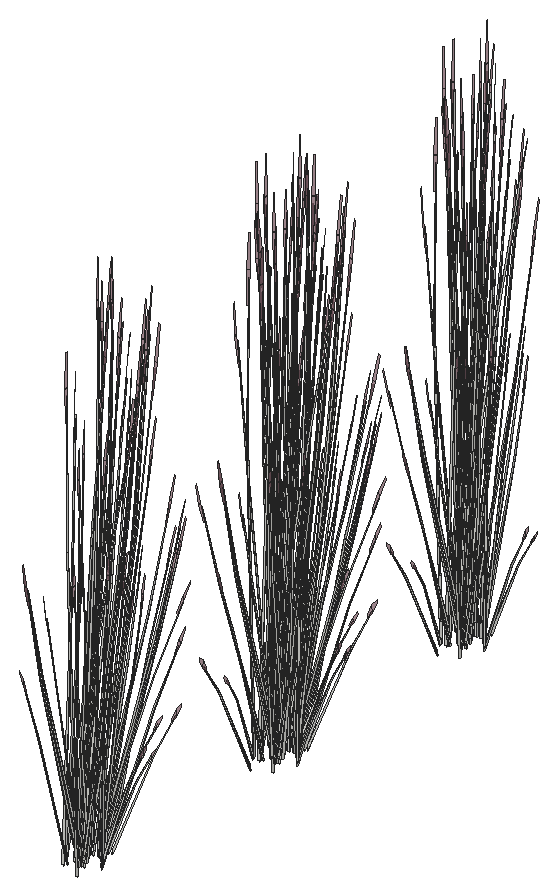
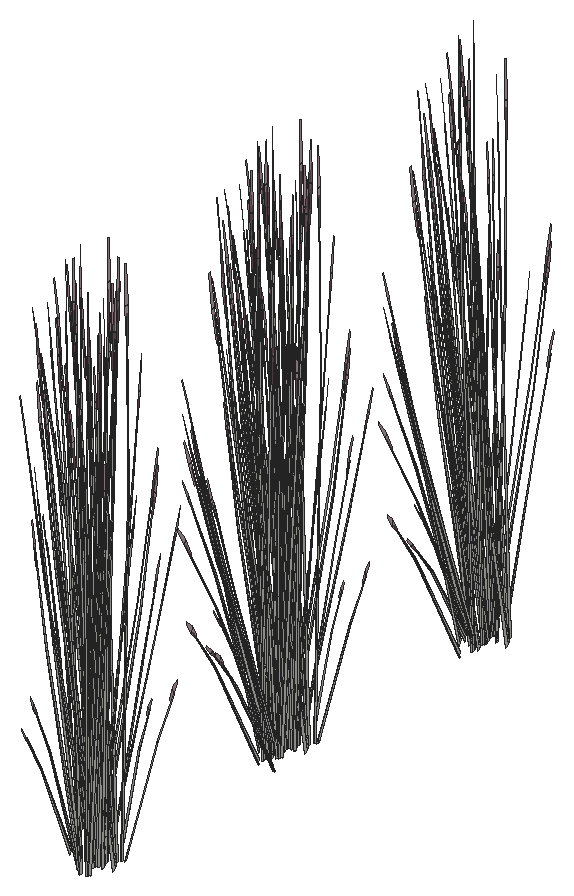
# SketchUp Ruby script. Lengths in inches.
U = 1.inch
M = Sketchup.active_model
def pt(a) = Geom::Point3d.new(a.map { |v| v * U })
def face(e, loops, mat)
  f = e.add_face(loops[0].map { |a| pt(a) })
  loops[1..].each { |l| e.add_face(l.map { |a| pt(a) }).erase! }
  f.material = f.back_material = mat if mat
  f
end
# faces: each face lists its corners as indices into pts; further lists are holes
def faces(e, pts, list, mat = nil) = list.each { |f| face(e, (f[0].is_a?(Array) ? f : [f]).map { |l| l.map { |i| pts[i] } }, mat) }
# xy, xz, yz: faces in a plane at the given z, y or x. An outline is a flat list of corners, or four numbers for a rectangle; further outlines are holes
def ring(l) = l.size == 4 ? [[l[0], l[1]], [l[2], l[1]], [l[2], l[3]], [l[0], l[3]]] : l.each_slice(2).to_a
def flat(e, list, mat, &to3) = list.each { |f| face(e, (f[0].is_a?(Array) ? f : [f]).map { |l| ring(l).map { |u, v| to3.(u, v) } }, mat) }
def xy(e, z, list, mat = nil) = flat(e, list, mat) { |x, y| [x, y, z] }
def xz(e, y, list, mat = nil) = flat(e, list, mat) { |x, z| [x, y, z] }
def yz(e, x, list, mat = nil) = flat(e, list, mat) { |y, z| [x, y, z] }
def lines(e, pts, list) = list.each { |a, b| e.add_line(pt(pts[a]), pt(pts[b])) }
# prism: a flat outline (further loops are holes) pulled along v
def prism(e, loops, v, mat = nil)
  f = face(e, loops, mat); d = Geom::Vector3d.new(v.map { |x| x * U })
  f.pushpull(f.normal.samedirection?(d) ? d.length : -d.length)
end
def box(e, o, s, mat = nil) = prism(e, [[o, [o[0] + s[0], o[1], o[2]], [o[0] + s[0], o[1] + s[1], o[2]], [o[0], o[1] + s[1], o[2]]]], [0, 0, s[2]], mat)
def at(x, y, z, deg = 0) = Geom::Transformation.translation(pt([x, y, z])) * Geom::Transformation.rotation(ORIGIN, Z_AXIS, deg.degrees)
def axes(o, x, y, z) = Geom::Transformation.new([*x, 0, *y, 0, *z, 0, *pt(o).to_a, 1])
def part(name) = M.definitions.add(name)
# library, detail: a bought-in or finely detailed component or shape, given as its bounding box
def library(name, o, s) = part(name).tap { |d| box(d.entities, o, s) }
def detail(e, o, s) = box(e.add_group.entities, o, s)
def put(e, d, t, mat = nil) = e.add_instance(d, t).tap { |i| i.material = mat if mat }
def group(e, t, mat = nil) = e.add_group.tap { |g| g.transformation = t; g.material = mat if mat }.entities
root = M.entities
M.materials.add("LightPink_Translucent").color = [144, 107, 117]
M.materials["LightPink_Translucent"].alpha = 0.75
c1 = part("blade")
p = [[2.15,0.21,22],[0,0.17,0],[0.09,0.45,0],[2.18,0.31,22],[2.29,0.31,22],[0.38,0.45,0],
  [2.48,0.24,33],[2.49,0.24,33],[2.48,0.22,33]]
faces(c1.entities,p,[[0,1,2,3],[4,5,2,3],[6,3,4,7],[8,0,3,6]])
c2 = part("seeds")
p = [[0.3,-0.1,1.38],[-0.01,-0.03,1.59],[-0.01,-0.03,0.03],[0.14,-0.07,-0.07],[0.29,-0.03,3],[0.15,0.01,3.11]]
faces(c2.entities,p,[[0,1,2,3],[1,0,4,5]],"LightPink_Translucent")
c3 = part("blade with seeds")
put(c3.entities,c1,at(0,0,0))
put(c3.entities,c2,axes([2.4,0.25,30.99],[1.5799,-0.05474,1.17369],[-0.12525,1.92788,0.29478],[-0.07173,-0.02425,1.56792]))
put(root,c3,axes([431.59,18.82,0.23],[-0.10696,0.11169,1.22981],[-0.32033,-0.19549,-0.26449],[0.05938,-0.24312,0.52581]))
put(root,c3,axes([431.85,19.65,2.28],[0.00979,-0.51041,-0.61099],[0.4123,0.03428,0.07373],[0.04351,-0.21623,0.8643]))
put(root,c3,axes([431.77,19.48,2.03],[-0.26937,-0.37076,-0.43945],[0.28456,-0.3247,-0.34039],[0.04099,-0.18838,0.84085]))
put(root,c3,axes([432.02,19.34,1.89],[0.2546,-0.29052,-0.30456],[0.24101,0.33173,0.39319],[0.03667,-0.16855,0.75234]))
put(root,c3,axes([432.34,19.17,-0.72],[-0.05632,-0.04347,1.51654],[-0.14467,-0.48565,-0.23168],[0.09759,-0.13179,0.25832]))
put(root,c3,axes([432.34,20.54,2.28],[0.19655,-0.43539,-0.61099],[0.34443,0.30942,0.07373],[0.11736,-0.15774,0.8643]))
put(root,c3,axes([432.33,20.33,2.03],[-0.09666,-0.50384,-0.43945],[0.36608,-0.08814,-0.34039],[0.10491,-0.13533,0.84085]))
put(root,c3,axes([430.53,19.18,-0.26],[0.35217,-0.2759,-0.427],[0.2105,0.49473,0],[0.08021,-0.06284,1.35453]))
put(root,c3,axes([432.625,20.14,0.23],[-0.13443,-0.01634,1.22981],[-0.13772,-0.43844,-0.26449],[0.16514,-0.12403,0.52581]))
put(root,c3,axes([430.95,20.31,-0.23],[0.25345,-0.41475,-0.53624],[0.31485,0.37608,-0.14074],[0.10156,-0.10346,1.18365]))
put(root,c3,axes([432.78,19.33,0.38],[-0.12533,0.28089,0.9878],[-0.10773,-0.37739,0.72577],[0.10352,-0.09457,0.21757]))
put(root,c3,axes([432.6,20.39,1.89],[0.32754,-0.07886,-0.30456],[0.08649,0.45081,0.39319],[0.09386,-0.12109,0.75234]))
put(root,c3,axes([430.68,20.8,0.29],[-0.04385,-0.62963,-0.25022],[0.45669,-0.03807,-0.43002],[0.08042,-0.08387,1.37348]))
put(root,c3,axes([430.62,19.4,-0.26],[0.35106,0.13653,-0.26641],[-0.08839,0.48081,0.26641],[0.07077,-0.05545,1.19518]))
put(root,c3,axes([432.5,21.45,2.03],[0.10194,-0.50193,-0.43945],[0.34951,0.17204,-0.34039],[0.14072,-0.04602,0.84085]))
put(root,c3,axes([431.95,19.41,0.04],[0.23526,-0.55293,0],[0.3936,0.30836,-0.44382],[0.08964,0.07023,1.40792]))
put(root,c3,axes([432.875,21.59,-0.3],[-0.24235,0.06622,1.21762],[-0.03858,-0.5271,0.0697],[0.16974,-0.07978,0.69287]))
put(root,c3,axes([433.31,21.125,-0.06],[-0.23329,-0.35284,-0.05579],[0.2555,-0.3233,-0.25298],[0.0724,-0.02276,0.83441]))
put(root,c3,axes([431.74,19.7,0.13],[-0.35217,-0.2759,0.427],[0.2105,-0.49473,0],[0.08021,0.06284,1.35453]))
put(root,c3,axes([432.43,21.63,2.28],[0.33065,-0.2437,-0.61099],[0.18427,0.50165,0.07373],[0.15976,-0.05699,0.8643]))
put(root,c3,axes([430.25,20.39,-0.63],[-0.37038,0.22092,1.10879],[-0.11789,-0.63387,0.43083],[0.22743,0.01055,1.26112]))
put(root,c3,axes([431.24,20.55,0.25],[0.07259,-0.49245,0.12452],[0.35466,0.08548,-0.35559],[0.06454,0.05057,1.09]))
put(root,c3,axes([433.14,21.25,-0.72],[-0.01967,-0.08377,1.51654],[0.1364,-0.49004,-0.23168],[0.13759,-0.00705,0.25832]))
put(root,c3,axes([431.09,20.68,0.34],[-0.22605,-0.46315,0.38476],[0.34239,-0.32614,-0.18517],[0.07315,0.05731,1.23533]))
put(root,c3,axes([431.2,20.71,0.29],[0.37992,-0.36634,-0.25022],[0.25264,0.51764,-0.43002],[0.09374,0.05257,1.37348]))
put(root,c3,axes([432.71,21.68,1.89],[0.31272,0.15393,-0.30456],[-0.09121,0.44909,0.39319],[0.1259,-0.04118,0.75234]))
put(root,c3,axes([432.16,19.74,-0.26],[0.35217,0.2759,-0.427],[-0.2105,0.49473,0],[0.08021,0.06284,1.35453]))
put(root,c3,axes([431.49,21.31,-0.1],[0.42099,0,0],[0,0.57126,0],[0,0,1.5343]))
put(root,c3,axes([432.0625,19.95,-0.26],[0.08839,0.48081,-0.26641],[-0.35106,0.13653,0.26641],[0.07077,0.05545,1.19518]))
put(root,c3,axes([431.36,21.02,0.05],[-0.4756,-0.11626,0.42311],[0.09679,-0.6566,0.16603],[0.0695,0.0634,1.46899]))
put(root,c3,axes([431.4375,22.58,-0.12],[0.39505,-0.18722,-0.1651],[0.13882,0.53931,0.00007],[0.04361,-0.02069,1.49552]))
put(root,c3,axes([431.48,21.56,-0.1],[0.26266,0.35642,0],[-0.26266,0.35642,0],[0,0,1.45569]))
put(root,c3,axes([431.65,20.8,-0.23],[0.39143,0.09047,-0.53624],[-0.0826,0.55804,-0.14074],[0.11681,0.06762,1.18365]))
put(root,c3,axes([433.38,21.77,0.38],[-0.23249,0.0911,0.9878],[0.10944,-0.37648,0.72577],[0.12334,0.02576,0.21757]))
put(root,c3,axes([431.48,21.14,0.34],[0.18257,-0.49721,0.38476],[0.37935,0.23929,-0.18517],[0,0.11462,1.23533]))
put(root,c3,axes([431.45,20.97,-0.1],[0.22605,0.46315,-0.38476],[-0.34239,0.32614,0.18517],[0.07315,0.05731,1.23533]))
put(root,c3,axes([432.4375,21.42,0.13],[0,-0.5518,0.427],[0.42099,0,0],[0,0.12568,1.35453]))
put(root,c3,axes([431.64,21.26,0.25],[0.35059,-0.16092,0.12452],[0.12277,0.45952,-0.35559],[0,0.10113,1.09]))
put(root,c3,axes([432.94,22.375,0.23],[-0.09062,-0.13571,1.22981],[0.11791,-0.44895,-0.26449],[0.18335,0.06082,0.52581]))
put(root,c3,axes([431.32,22.87,-0.1],[0.37935,0.24773,0],[-0.18257,0.51475,0],[0,0,1.5046]))
put(root,c3,axes([432.11,22.65,2.28],[0.37615,0.01329,-0.61099],[-0.02526,0.55946,0.07373],[0.15935,0.05904,0.8643]))
put(root,c3,axes([432.72,21.51,0.04],[0.47052,0,0],[0,0.61671,-0.44382],[0,0.14046,1.40792]))
put(root,c3,axes([431.52,21.29,0.29],[0.42377,0.26329,-0.25022],[-0.20405,0.55571,-0.43002],[0.01332,0.13644,1.37348]))
put(root,c3,axes([432.34,22.88,1.89],[0.2141,0.34548,-0.30456],[-0.24447,0.32704,0.39319],[0.12421,0.04976,0.75234]))
put(root,c3,axes([432.4375,21.92,-0.26],[-0.26266,0.34428,-0.26641],[-0.26266,-0.34428,0.26641],[0,0.11089,1.19518]))
put(root,c3,axes([432.62,21.93,-0.26],[0,0.5518,-0.427],[-0.42099,0,0],[0,0.12568,1.35453]))
put(root,c3,axes([432.08,23.08,0.38],[-0.21187,-0.15866,0.9878],[0.27357,-0.16121,0.72577],[0.07379,0.13656,0.21757]))
put(root,c3,axes([432.14,23.67,-0.72],[0.02741,-0.07966,1.51654],[0.34514,-0.23462,-0.23168],[0.10464,0.12143,0.25832]))
put(root,c3,axes([431.6875,21.86,-0.2],[0.13798,0.50522,-0.59522],[-0.39745,0.18195,-0.15622],[0.01525,0.17108,1.31385]))
put(root,c3,axes([431.61,23.3,2.03],[0.37131,-0.13117,-0.43945],[0.06495,0.49674,-0.34039],[0.09973,0.14235,0.84085]))
put(root,c3,axes([432.12,23.8,0.29],[-0.2413,-0.01731,0.90352],[0.15935,-0.36755,0.49885],[0.09532,0.13058,0.70873]))
put(root,c3,axes([431.33,22.91,0.23],[0.00664,-0.18292,1.22981],[0.31732,-0.20432,-0.26449],[0.09796,0.21893,0.52581]))
put(root,c3,axes([430.78,23.53,2.03],[0.3699,0.13833,-0.43945],[-0.12679,0.47426,-0.34039],[0.03392,0.19095,0.84085]))
put(root,c3,axes([433.22,41.86,0.23],[-0.10696,0.11169,1.22981],[-0.32033,-0.19549,-0.26449],[0.05938,-0.24312,0.52581]))
put(root,c3,axes([432.43,41.26,-0.72],[-0.06312,0.01988,1.51654],[-0.34903,-0.22379,-0.23168],[0.00586,-0.18666,0.25832]))
put(root,c3,axes([433.48,42.69,2.28],[0.00979,-0.51041,-0.61099],[0.4123,0.03428,0.07373],[0.04351,-0.21623,0.8643]))
put(root,c3,axes([432.77,41.87,1.89],[0.11344,-0.42434,-0.30456],[0.33096,0.12377,0.39319],[-0.03035,-0.17085,0.75234]))
put(root,c3,axes([432.83,40.97,0.38],[0.04827,0.32177,0.9878],[-0.26778,-0.17821,0.72577],[0.02882,-0.16476,0.21757]))
put(root,c3,axes([433.4,42.52,2.03],[-0.26937,-0.37076,-0.43945],[0.28456,-0.3247,-0.34039],[0.04099,-0.18838,0.84085]))
put(root,c3,axes([433.65,42.38,1.89],[0.2546,-0.29052,-0.30456],[0.24101,0.33173,0.39319],[0.03667,-0.16855,0.75234]))
put(root,c3,axes([433.97,42.21,-0.72],[-0.05632,-0.04347,1.51654],[-0.14467,-0.48565,-0.23168],[0.09759,-0.13179,0.25832]))
put(root,c3,axes([433.97,43.58,2.28],[0.19655,-0.43539,-0.61099],[0.34443,0.30942,0.07373],[0.11736,-0.15774,0.8643]))
put(root,c3,axes([431.84,42.31,0.04],[-0.23526,-0.55293,0],[0.3936,-0.30836,-0.44382],[0.08964,-0.07023,1.40792]))
put(root,c3,axes([433.96,43.375,2.03],[-0.09666,-0.50384,-0.43945],[0.36608,-0.08814,-0.34039],[0.10491,-0.13533,0.84085]))
put(root,c3,axes([432.16,42.22,-0.26],[0.35217,-0.2759,-0.427],[0.2105,0.49473,0],[0.08021,-0.06284,1.35453]))
put(root,c3,axes([434.25,43.18,0.23],[-0.13443,-0.01634,1.22981],[-0.13772,-0.43844,-0.26449],[0.16514,-0.12403,0.52581]))
put(root,c3,axes([432.58,43.36,-0.23],[0.25345,-0.41475,-0.53624],[0.31485,0.37608,-0.14074],[0.10156,-0.10346,1.18365]))
put(root,c3,axes([434.41,42.37,0.38],[-0.12533,0.28089,0.9878],[-0.10773,-0.37739,0.72577],[0.10352,-0.09457,0.21757]))
put(root,c3,axes([434.23,43.43,1.89],[0.32754,-0.07886,-0.30456],[0.08649,0.45081,0.39319],[0.09386,-0.12109,0.75234]))
put(root,c3,axes([432.14,44.08,-0.1],[0.18257,-0.49721,-0.38476],[0.37935,0.23929,0.18517],[0,-0.11462,1.23533]))
put(root,c3,axes([432.31,43.84,0.29],[-0.04385,-0.62963,-0.25022],[0.45669,-0.03807,-0.43002],[0.08042,-0.08387,1.37348]))
put(root,c3,axes([432.25,42.44,-0.26],[0.35106,0.13653,-0.26641],[-0.08839,0.48081,0.26641],[0.07077,-0.05545,1.19518]))
put(root,c3,axes([432.37,44.33,0.09],[0.42398,0.26744,0.20696],[-0.20405,0.55571,0.43002],[0,-0.1281,1.38067]))
put(root,c3,axes([432.23,43.96,0.34],[-0.40861,0.03406,0.38476],[-0.03695,-0.56543,-0.18517],[0.07315,-0.05731,1.23533]))
put(root,c3,axes([434.13,44.49,2.03],[0.10194,-0.50193,-0.43945],[0.34951,0.17204,-0.34039],[0.14072,-0.04602,0.84085]))
put(root,c3,axes([433.58,42.45,0.04],[0.23526,-0.55293,0],[0.3936,0.30836,-0.44382],[0.08964,0.07023,1.40792]))
put(root,c3,axes([432.22,44.16,0.03],[0.1636,0.61702,0.39349],[-0.46745,0.21456,0.15441],[0.00571,-0.11338,1.36617]))
put(root,c3,axes([434.5,44.63,-0.3],[-0.24235,0.06622,1.21762],[-0.03858,-0.5271,0.0697],[0.16974,-0.07978,0.69287]))
put(root,c3,axes([434.94,44.17,-0.06],[-0.23329,-0.35284,-0.05579],[0.2555,-0.3233,-0.25298],[0.0724,-0.02276,0.83441]))
put(root,c3,axes([432.8,44.21,-0.1],[0,-0.63847,0],[0.47052,0,0],[0,0,1.54332]))
put(root,c3,axes([433.375,42.74,0.13],[-0.35217,-0.2759,0.427],[0.2105,-0.49473,0],[0.08021,0.06284,1.35453]))
put(root,c3,axes([434.0625,44.68,2.28],[0.33065,-0.2437,-0.61099],[0.18427,0.50165,0.07373],[0.15976,-0.05699,0.8643]))
put(root,c3,axes([432.58,43.8125,0.03],[-0.312,0.50076,0.39349],[-0.37066,-0.44204,0.15441],[0.07522,-0.04998,1.36617]))
put(root,c3,axes([432.92,44.71,-0.02],[-0.35001,-0.47494,-0.05273],[0.35022,-0.47523,0],[-0.01222,-0.01659,1.50991]))
put(root,c3,axes([432.04,42.99,0.13],[-0.1087,0.54839,0.15172],[-0.39778,-0.15519,0.30174],[0.06871,-0.00267,1.3795]))
put(root,c3,axes([431.875,43.43,-0.63],[-0.37038,0.22092,1.10879],[-0.11789,-0.63387,0.43083],[0.22743,0.01055,1.26112]))
put(root,c3,axes([432.87,43.6,0.25],[0.07259,-0.49245,0.12452],[0.35466,0.08548,-0.35559],[0.06454,0.05057,1.09]))
put(root,c3,axes([434.77,44.29,-0.72],[-0.01967,-0.08377,1.51654],[0.1364,-0.49004,-0.23168],[0.13759,-0.00705,0.25832]))
put(root,c3,axes([432.72,43.73,0.34],[-0.22605,-0.46315,0.38476],[0.34239,-0.32614,-0.18517],[0.07315,0.05731,1.23533]))
put(root,c3,axes([432,45.82,0.13],[0.40434,-0.14646,0.15172],[0.09984,0.54504,0.30174],[-0.03606,-0.07941,1.3795]))
put(root,c3,axes([432.83,43.76,0.29],[0.37992,-0.36634,-0.25022],[0.25264,0.51764,-0.43002],[0.09374,0.05257,1.37348]))
put(root,c3,axes([434.34,44.72,1.89],[0.31272,0.15393,-0.30456],[-0.09121,0.44909,0.39319],[0.1259,-0.04118,0.75234]))
put(root,c3,axes([433.79,42.78,-0.26],[0.35217,0.2759,-0.427],[-0.2105,0.49473,0],[0.08021,0.06284,1.35453]))
put(root,c3,axes([433.12,44.36,-0.1],[0.42099,0,0],[0,0.57126,0],[0,0,1.5343]))
put(root,c3,axes([433.24,43.02,0.13],[-0.40434,0.14646,0.15172],[-0.09984,-0.54504,0.30174],[0.03606,0.07941,1.3795]))
put(root,c3,axes([433.69,42.99,-0.26],[0.08839,0.48081,-0.26641],[-0.35106,0.13653,0.26641],[0.07077,0.05545,1.19518]))
put(root,c3,axes([432.99,44.07,0.05],[-0.4756,-0.11626,0.42311],[0.09679,-0.6566,0.16603],[0.0695,0.0634,1.46899]))
put(root,c3,axes([432.61,45.6875,-0.1],[-0.12277,-0.47573,0],[0.35059,-0.1666,0],[0,0,1.32759]))
put(root,c3,axes([433.07,45.62,-0.12],[0.39505,-0.18722,-0.1651],[0.13882,0.53931,0.00007],[0.04361,-0.02069,1.49552]))
put(root,c3,axes([433.2,45.85,0.13],[0.1087,-0.54839,0.15172],[0.39778,0.15519,0.30174],[-0.06871,0.00267,1.3795]))
put(root,c3,axes([433.11,44.6,-0.1],[0.26266,0.35642,0],[-0.26266,0.35642,0],[0,0,1.45569]))
put(root,c3,axes([433.82,44.45,0.13],[-0.29564,-0.40194,0.15172],[0.29793,-0.38985,0.30174],[-0.03265,0.08208,1.3795]))
put(root,c3,axes([433.28,43.84,-0.23],[0.39143,0.09047,-0.53624],[-0.0826,0.55804,-0.14074],[0.11681,0.06762,1.18365]))
put(root,c3,axes([435.01,44.8125,0.38],[-0.23249,0.0911,0.9878],[0.10944,-0.37648,0.72577],[0.12334,0.02576,0.21757]))
put(root,c3,axes([432.52,45.9,-0.11],[-0.37935,-0.24773,0],[0.18257,-0.51475,0],[0,0,1.39928]))
put(root,c3,axes([433.11,44.18,0.34],[0.18257,-0.49721,0.38476],[0.37935,0.23929,-0.18517],[0,0.11462,1.23533]))
put(root,c3,axes([433.04,44.47,-0.03],[0,0.63816,-0.04848],[-0.47052,0,0],[0,0.02005,1.54256]))
put(root,c3,axes([433.07,44.02,-0.1],[0.22605,0.46315,-0.38476],[-0.34239,0.32614,0.18517],[0.07315,0.05731,1.23533]))
put(root,c3,axes([434.07,44.46,0.13],[0,-0.5518,0.427],[0.42099,0,0],[0,0.12568,1.35453]))
put(root,c3,axes([433.01,44.875,0.34],[0.40861,-0.03406,0.38476],[0.03695,0.56543,-0.18517],[-0.07315,0.05731,1.23533]))
put(root,c3,axes([433.27,44.3,0.25],[0.35059,-0.16092,0.12452],[0.12277,0.45952,-0.35559],[0,0.10113,1.09]))
put(root,c3,axes([434.57,45.42,0.23],[-0.09062,-0.13571,1.22981],[0.11791,-0.44895,-0.26449],[0.18335,0.06082,0.52581]))
put(root,c3,axes([432.95,45.91,-0.1],[0.37935,0.24773,0],[-0.18257,0.51475,0],[0,0,1.5046]))
put(root,c3,axes([433.02,45.12,0.25],[0.278,0.33153,0.12452],[-0.23189,0.37404,-0.35559],[-0.06454,0.05057,1.09]))
put(root,c3,axes([433.74,45.69,2.28],[0.37615,0.01329,-0.61099],[-0.02526,0.55946,0.07373],[0.15935,0.05904,0.8643]))
put(root,c3,axes([433.32,46.14,0.13],[0.35217,-0.2759,0.427],[0.2105,0.49473,0],[-0.08021,0.06284,1.35453]))
put(root,c3,axes([432.81,45.7,-0.03],[0.1636,0.63392,-0.05171],[-0.46745,0.22213,0],[0.00571,0.02214,1.48069]))
put(root,c3,axes([434.35,44.56,0.04],[0.47052,0,0],[0,0.61671,-0.44382],[0,0.14046,1.40792]))
put(root,c3,axes([434.17,44.87,-0.11],[-0.47029,-0.00441,-0.0428],[0,-0.61671,0.42951],[-0.01478,0.14039,1.36183]))
put(root,c3,axes([433.15,44.34,0.29],[0.42377,0.26329,-0.25022],[-0.20405,0.55571,-0.43002],[0.01332,0.13644,1.37348]))
put(root,c3,axes([433.97,45.92,1.89],[0.2141,0.34548,-0.30456],[-0.24447,0.32704,0.39319],[0.12421,0.04976,0.75234]))
put(root,c3,axes([434.07,44.96,-0.26],[-0.26266,0.34428,-0.26641],[-0.26266,-0.34428,0.26641],[0,0.11089,1.19518]))
put(root,c3,axes([433.1,44.75,-0.1],[-0.18257,0.49721,-0.38476],[-0.37935,-0.23929,0.18517],[0,0.11462,1.23533]))
put(root,c3,axes([433.11,46.17,0],[0.47108,0.17935,0.2645],[-0.11785,0.64108,-0.31383],[-0.07797,0.08023,1.41801]))
put(root,c3,axes([434.25,44.97,-0.26],[0,0.5518,-0.427],[-0.42099,0,0],[0,0.12568,1.35453]))
put(root,c3,axes([433.71,46.12,0.38],[-0.21187,-0.15866,0.9878],[0.27357,-0.16121,0.72577],[0.07379,0.13656,0.21757]))
put(root,c3,axes([433.4,46.52,0.04],[0.23526,0.55293,0],[-0.3936,0.30836,-0.44382],[-0.08964,0.07023,1.40792]))
put(root,c3,axes([433.77,46.71,-0.72],[0.02741,-0.07966,1.51654],[0.34514,-0.23462,-0.23168],[0.10464,0.12143,0.25832]))
put(root,c3,axes([433.32,44.9,-0.2],[0.13798,0.50522,-0.59522],[-0.39745,0.18195,-0.15622],[0.01525,0.17108,1.31385]))
put(root,c3,axes([433.24,46.34,2.03],[0.37131,-0.13117,-0.43945],[0.06495,0.49674,-0.34039],[0.09973,0.14235,0.84085]))
put(root,c3,axes([433.75,46.84,0.29],[-0.2413,-0.01731,0.90352],[0.15935,-0.36755,0.49885],[0.09532,0.13058,0.70873]))
put(root,c3,axes([432.96,45.95,0.23],[0.00664,-0.18292,1.22981],[0.31732,-0.20432,-0.26449],[0.09796,0.21893,0.52581]))
put(root,c3,axes([432.16,46.69,-0.72],[0.0609,-0.03003,1.51654],[0.36632,0.16527,-0.23168],[0.01071,0.18627,0.25832]))
put(root,c3,axes([432.41,46.57,2.03],[0.3699,0.13833,-0.43945],[-0.12679,0.47426,-0.34039],[0.03392,0.19095,0.84085]))
put(root,c3,axes([432.24,46.86,1.89],[-0.11344,0.42434,-0.30456],[-0.33096,-0.12377,0.39319],[0.03035,0.17085,0.75234]))
put(root,c3,axes([432.28,46.48,2.28],[0.17959,0.44867,-0.61099],[-0.36969,0.25004,0.07373],[0.042,0.21679,0.8643]))
put(root,c3,axes([433.22,65.86,0.23],[-0.10696,0.11169,1.22981],[-0.32033,-0.19549,-0.26449],[0.05938,-0.24312,0.52581]))
put(root,c3,axes([432.43,65.26,-0.72],[-0.06312,0.01988,1.51654],[-0.34903,-0.22379,-0.23168],[0.00586,-0.18666,0.25832]))
put(root,c3,axes([433.48,66.69,2.28],[0.00979,-0.51041,-0.61099],[0.4123,0.03428,0.07373],[0.04351,-0.21623,0.8643]))
put(root,c3,axes([432.77,65.87,1.89],[0.11344,-0.42434,-0.30456],[0.33096,0.12377,0.39319],[-0.03035,-0.17085,0.75234]))
put(root,c3,axes([432.83,64.97,0.38],[0.04827,0.32177,0.9878],[-0.26778,-0.17821,0.72577],[0.02882,-0.16476,0.21757]))
put(root,c3,axes([433.4,66.52,2.03],[-0.26937,-0.37076,-0.43945],[0.28456,-0.3247,-0.34039],[0.04099,-0.18838,0.84085]))
put(root,c3,axes([433.65,66.38,1.89],[0.2546,-0.29052,-0.30456],[0.24101,0.33173,0.39319],[0.03667,-0.16855,0.75234]))
put(root,c3,axes([433.97,66.21,-0.72],[-0.05632,-0.04347,1.51654],[-0.14467,-0.48565,-0.23168],[0.09759,-0.13179,0.25832]))
put(root,c3,axes([433.97,67.58,2.28],[0.19655,-0.43539,-0.61099],[0.34443,0.30942,0.07373],[0.11736,-0.15774,0.8643]))
put(root,c3,axes([431.84,66.31,0.04],[-0.23526,-0.55293,0],[0.3936,-0.30836,-0.44382],[0.08964,-0.07023,1.40792]))
put(root,c3,axes([433.96,67.375,2.03],[-0.09666,-0.50384,-0.43945],[0.36608,-0.08814,-0.34039],[0.10491,-0.13533,0.84085]))
put(root,c3,axes([432.16,66.22,-0.26],[0.35217,-0.2759,-0.427],[0.2105,0.49473,0],[0.08021,-0.06284,1.35453]))
put(root,c3,axes([434.25,67.18,0.23],[-0.13443,-0.01634,1.22981],[-0.13772,-0.43844,-0.26449],[0.16514,-0.12403,0.52581]))
put(root,c3,axes([432.58,67.36,-0.23],[0.25345,-0.41475,-0.53624],[0.31485,0.37608,-0.14074],[0.10156,-0.10346,1.18365]))
put(root,c3,axes([434.41,66.37,0.38],[-0.12533,0.28089,0.9878],[-0.10773,-0.37739,0.72577],[0.10352,-0.09457,0.21757]))
put(root,c3,axes([434.23,67.43,1.89],[0.32754,-0.07886,-0.30456],[0.08649,0.45081,0.39319],[0.09386,-0.12109,0.75234]))
put(root,c3,axes([432.14,68.08,-0.1],[0.18257,-0.49721,-0.38476],[0.37935,0.23929,0.18517],[0,-0.11462,1.23533]))
put(root,c3,axes([432.31,67.84,0.29],[-0.04385,-0.62963,-0.25022],[0.45669,-0.03807,-0.43002],[0.08042,-0.08387,1.37348]))
put(root,c3,axes([432.25,66.44,-0.26],[0.35106,0.13653,-0.26641],[-0.08839,0.48081,0.26641],[0.07077,-0.05545,1.19518]))
put(root,c3,axes([432.37,68.33,0.09],[0.42398,0.26744,0.20696],[-0.20405,0.55571,0.43002],[0,-0.1281,1.38067]))
put(root,c3,axes([432.23,67.96,0.34],[-0.40861,0.03406,0.38476],[-0.03695,-0.56543,-0.18517],[0.07315,-0.05731,1.23533]))
put(root,c3,axes([434.13,68.49,2.03],[0.10194,-0.50193,-0.43945],[0.34951,0.17204,-0.34039],[0.14072,-0.04602,0.84085]))
put(root,c3,axes([433.58,66.45,0.04],[0.23526,-0.55293,0],[0.3936,0.30836,-0.44382],[0.08964,0.07023,1.40792]))
put(root,c3,axes([432.22,68.16,0.03],[0.1636,0.61702,0.39349],[-0.46745,0.21456,0.15441],[0.00571,-0.11338,1.36617]))
put(root,c3,axes([434.5,68.63,-0.3],[-0.24235,0.06622,1.21762],[-0.03858,-0.5271,0.0697],[0.16974,-0.07978,0.69287]))
put(root,c3,axes([434.94,68.17,-0.06],[-0.23329,-0.35284,-0.05579],[0.2555,-0.3233,-0.25298],[0.0724,-0.02276,0.83441]))
put(root,c3,axes([432.8,68.21,-0.1],[0,-0.63847,0],[0.47052,0,0],[0,0,1.54332]))
put(root,c3,axes([433.375,66.74,0.13],[-0.35217,-0.2759,0.427],[0.2105,-0.49473,0],[0.08021,0.06284,1.35453]))
put(root,c3,axes([434.0625,68.68,2.28],[0.33065,-0.2437,-0.61099],[0.18427,0.50165,0.07373],[0.15976,-0.05699,0.8643]))
put(root,c3,axes([432.58,67.8125,0.03],[-0.312,0.50076,0.39349],[-0.37066,-0.44204,0.15441],[0.07522,-0.04998,1.36617]))
put(root,c3,axes([432.92,68.71,-0.02],[-0.35001,-0.47494,-0.05273],[0.35022,-0.47523,0],[-0.01222,-0.01659,1.50991]))
put(root,c3,axes([432.04,66.99,0.13],[-0.1087,0.54839,0.15172],[-0.39778,-0.15519,0.30174],[0.06871,-0.00267,1.3795]))
put(root,c3,axes([431.875,67.43,-0.63],[-0.37038,0.22092,1.10879],[-0.11789,-0.63387,0.43083],[0.22743,0.01055,1.26112]))
put(root,c3,axes([432.87,67.6,0.25],[0.07259,-0.49245,0.12452],[0.35466,0.08548,-0.35559],[0.06454,0.05057,1.09]))
put(root,c3,axes([434.77,68.29,-0.72],[-0.01967,-0.08377,1.51654],[0.1364,-0.49004,-0.23168],[0.13759,-0.00705,0.25832]))
put(root,c3,axes([432.72,67.73,0.34],[-0.22605,-0.46315,0.38476],[0.34239,-0.32614,-0.18517],[0.07315,0.05731,1.23533]))
put(root,c3,axes([432,69.82,0.13],[0.40434,-0.14646,0.15172],[0.09984,0.54504,0.30174],[-0.03606,-0.07941,1.3795]))
put(root,c3,axes([432.83,67.76,0.29],[0.37992,-0.36634,-0.25022],[0.25264,0.51764,-0.43002],[0.09374,0.05257,1.37348]))
put(root,c3,axes([434.34,68.72,1.89],[0.31272,0.15393,-0.30456],[-0.09121,0.44909,0.39319],[0.1259,-0.04118,0.75234]))
put(root,c3,axes([433.79,66.78,-0.26],[0.35217,0.2759,-0.427],[-0.2105,0.49473,0],[0.08021,0.06284,1.35453]))
put(root,c3,axes([433.12,68.36,-0.1],[0.42099,0,0],[0,0.57126,0],[0,0,1.5343]))
put(root,c3,axes([433.24,67.02,0.13],[-0.40434,0.14646,0.15172],[-0.09984,-0.54504,0.30174],[0.03606,0.07941,1.3795]))
put(root,c3,axes([433.69,66.99,-0.26],[0.08839,0.48081,-0.26641],[-0.35106,0.13653,0.26641],[0.07077,0.05545,1.19518]))
put(root,c3,axes([432.99,68.07,0.05],[-0.4756,-0.11626,0.42311],[0.09679,-0.6566,0.16603],[0.0695,0.0634,1.46899]))
put(root,c3,axes([432.61,69.6875,-0.1],[-0.12277,-0.47573,0],[0.35059,-0.1666,0],[0,0,1.32759]))
put(root,c3,axes([433.07,69.62,-0.12],[0.39505,-0.18722,-0.1651],[0.13882,0.53931,0.00007],[0.04361,-0.02069,1.49552]))
put(root,c3,axes([433.2,69.85,0.13],[0.1087,-0.54839,0.15172],[0.39778,0.15519,0.30174],[-0.06871,0.00267,1.3795]))
put(root,c3,axes([433.11,68.6,-0.1],[0.26266,0.35642,0],[-0.26266,0.35642,0],[0,0,1.45569]))
put(root,c3,axes([433.82,68.45,0.13],[-0.29564,-0.40194,0.15172],[0.29793,-0.38985,0.30174],[-0.03265,0.08208,1.3795]))
put(root,c3,axes([433.28,67.84,-0.23],[0.39143,0.09047,-0.53624],[-0.0826,0.55804,-0.14074],[0.11681,0.06762,1.18365]))
put(root,c3,axes([435.01,68.8125,0.38],[-0.23249,0.0911,0.9878],[0.10944,-0.37648,0.72577],[0.12334,0.02576,0.21757]))
put(root,c3,axes([432.52,69.9,-0.11],[-0.37935,-0.24773,0],[0.18257,-0.51475,0],[0,0,1.39928]))
put(root,c3,axes([433.11,68.18,0.34],[0.18257,-0.49721,0.38476],[0.37935,0.23929,-0.18517],[0,0.11462,1.23533]))
put(root,c3,axes([433.04,68.47,-0.03],[0,0.63816,-0.04848],[-0.47052,0,0],[0,0.02005,1.54256]))
put(root,c3,axes([433.07,68.02,-0.1],[0.22605,0.46315,-0.38476],[-0.34239,0.32614,0.18517],[0.07315,0.05731,1.23533]))
put(root,c3,axes([434.07,68.46,0.13],[0,-0.5518,0.427],[0.42099,0,0],[0,0.12568,1.35453]))
put(root,c3,axes([433.01,68.875,0.34],[0.40861,-0.03406,0.38476],[0.03695,0.56543,-0.18517],[-0.07315,0.05731,1.23533]))
put(root,c3,axes([433.27,68.3,0.25],[0.35059,-0.16092,0.12452],[0.12277,0.45952,-0.35559],[0,0.10113,1.09]))
